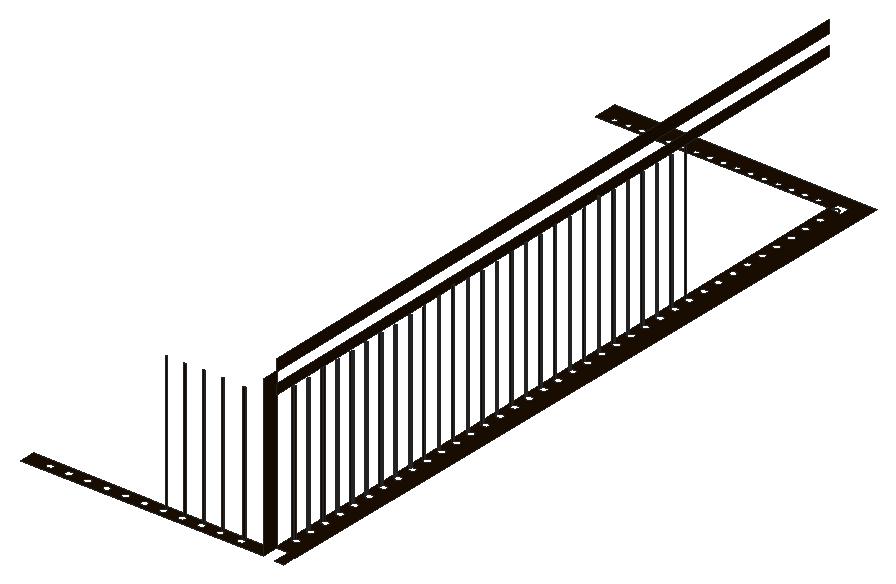
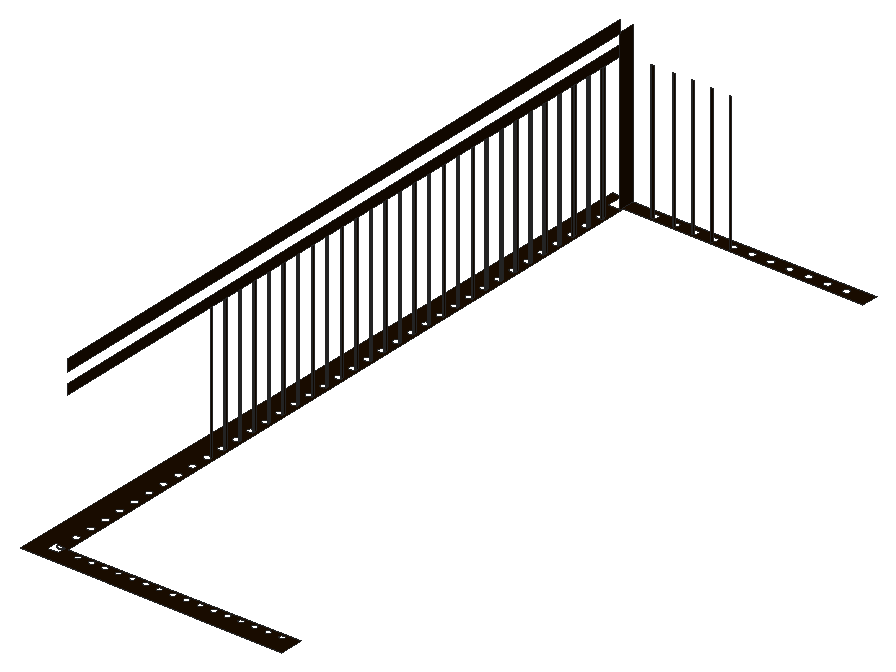
# SketchUp Ruby script. Lengths in inches.
U = 1.inch
M = Sketchup.active_model
def pt(a) = Geom::Point3d.new(a.map { |v| v * U })
def face(e, loops, mat)
  f = e.add_face(loops[0].map { |a| pt(a) })
  loops[1..].each { |l| e.add_face(l.map { |a| pt(a) }).erase! }
  f.material = f.back_material = mat if mat
  f
end
# faces: each face lists its corners as indices into pts; further lists are holes
def faces(e, pts, list, mat = nil) = list.each { |f| face(e, (f[0].is_a?(Array) ? f : [f]).map { |l| l.map { |i| pts[i] } }, mat) }
# xy, xz, yz: faces in a plane at the given z, y or x. An outline is a flat list of corners, or four numbers for a rectangle; further outlines are holes
def ring(l) = l.size == 4 ? [[l[0], l[1]], [l[2], l[1]], [l[2], l[3]], [l[0], l[3]]] : l.each_slice(2).to_a
def flat(e, list, mat, &to3) = list.each { |f| face(e, (f[0].is_a?(Array) ? f : [f]).map { |l| ring(l).map { |u, v| to3.(u, v) } }, mat) }
def xy(e, z, list, mat = nil) = flat(e, list, mat) { |x, y| [x, y, z] }
def xz(e, y, list, mat = nil) = flat(e, list, mat) { |x, z| [x, y, z] }
def yz(e, x, list, mat = nil) = flat(e, list, mat) { |y, z| [x, y, z] }
def lines(e, pts, list) = list.each { |a, b| e.add_line(pt(pts[a]), pt(pts[b])) }
# prism: a flat outline (further loops are holes) pulled along v
def prism(e, loops, v, mat = nil)
  f = face(e, loops, mat); d = Geom::Vector3d.new(v.map { |x| x * U })
  f.pushpull(f.normal.samedirection?(d) ? d.length : -d.length)
end
def box(e, o, s, mat = nil) = prism(e, [[o, [o[0] + s[0], o[1], o[2]], [o[0] + s[0], o[1] + s[1], o[2]], [o[0], o[1] + s[1], o[2]]]], [0, 0, s[2]], mat)
def at(x, y, z, deg = 0) = Geom::Transformation.translation(pt([x, y, z])) * Geom::Transformation.rotation(ORIGIN, Z_AXIS, deg.degrees)
def axes(o, x, y, z) = Geom::Transformation.new([*x, 0, *y, 0, *z, 0, *pt(o).to_a, 1])
def part(name) = M.definitions.add(name)
# library, detail: a bought-in or finely detailed component or shape, given as its bounding box
def library(name, o, s) = part(name).tap { |d| box(d.entities, o, s) }
def detail(e, o, s) = box(e.add_group.entities, o, s)
def put(e, d, t, mat = nil) = e.add_instance(d, t).tap { |i| i.material = mat if mat }
def group(e, t, mat = nil) = e.add_group.tap { |g| g.transformation = t; g.material = mat if mat }.entities
root = M.entities
M.materials.add("[Metal Seamed]1").color = [28, 14, 0]
xy(root,618.25,[[[275.92,67.28,361.97,67.28,361.97,73.28,366.15,73.28,366.15,67.28,369.3125,67.28,369.3125,72.19,369.37,72.19,372.33,325.44,278.88,326.53,278.8125,320.82,278.79,318.92,278.78,318.35,361.23,318.35,361.23,72.29,275.92,73.28],[361.98,317.52,366.15,321.28],[284.2,68.79,283.86,68.83,283.54,68.97,283.27,69.17,283.0625,69.45,282.93,69.76,282.89,70.1,282.93,70.44,283.0625,70.76,283.27,71.03,283.54,71.24,283.86,71.37,284.2,71.41,284.54,71.37,284.86,71.24,285.13,71.03,285.34,70.76,285.47,70.44,285.51,70.1,285.47,69.76,285.34,69.45,285.13,69.17,284.86,68.97,284.54,68.83],[351.89,68.79,351.55,68.83,351.23,68.97,350.96,69.17,350.75,69.45,350.62,69.76,350.58,70.1,350.62,70.44,350.75,70.76,350.96,71.03,351.23,71.24,351.55,71.37,351.89,71.41,352.23,71.37,352.55,71.24,352.82,71.03,353.03,70.76,353.16,70.44,353.2,70.1,353.16,69.76,353.03,69.45,352.82,69.17,352.55,68.97,352.23,68.83],[344.39,68.79,344.05,68.83,343.73,68.97,343.46,69.17,343.25,69.45,343.12,69.76,343.07,70.1,343.12,70.44,343.25,70.76,343.46,71.03,343.73,71.24,344.05,71.37,344.39,71.41,344.73,71.37,345.04,71.24,345.31,71.03,345.52,70.76,345.65,70.44,345.7,70.1,345.65,69.76,345.52,69.45,345.31,69.17,345.04,68.97,344.73,68.83],[337.7,68.79,337.36,68.83,337.04,68.97,336.77,69.17,336.5625,69.45,336.43,69.76,336.39,70.1,336.43,70.44,336.5625,70.76,336.77,71.03,337.04,71.24,337.36,71.37,337.7,71.41,338.04,71.37,338.36,71.24,338.63,71.03,338.84,70.76,338.97,70.44,339.01,70.1,338.97,69.76,338.84,69.45,338.63,69.17,338.36,68.97,338.04,68.83],[331.01,68.79,330.67,68.83,330.36,68.97,330.08,69.17,329.875,69.45,329.74,69.76,329.7,70.1,329.74,70.44,329.875,70.76,330.08,71.03,330.36,71.24,330.67,71.37,331.01,71.41,331.35,71.37,331.67,71.24,331.94,71.03,332.15,70.76,332.28,70.44,332.32,70.1,332.28,69.76,332.15,69.45,331.94,69.17,331.67,68.97,331.35,68.83],[324.32,68.79,323.98,68.83,323.67,68.97,323.4,69.17,323.1875,69.45,323.06,69.76,323.01,70.1,323.06,70.44,323.1875,70.76,323.4,71.03,323.67,71.24,323.98,71.37,324.32,71.41,324.66,71.37,324.98,71.24,325.25,71.03,325.46,70.76,325.59,70.44,325.64,70.1,325.59,69.76,325.46,69.45,325.25,69.17,324.98,68.97,324.66,68.83],[317.64,68.79,317.3,68.83,316.98,68.97,316.71,69.17,316.5,69.45,316.37,69.76,316.32,70.1,316.37,70.44,316.5,70.76,316.71,71.03,316.98,71.24,317.3,71.37,317.64,71.41,317.98,71.37,318.29,71.24,318.56,71.03,318.77,70.76,318.9,70.44,318.95,70.1,318.9,69.76,318.77,69.45,318.56,69.17,318.29,68.97,317.98,68.83],[310.95,68.79,310.61,68.83,310.29,68.97,310.02,69.17,309.8125,69.45,309.68,69.76,309.64,70.1,309.68,70.44,309.8125,70.76,310.02,71.03,310.29,71.24,310.61,71.37,310.95,71.41,311.29,71.37,311.61,71.24,311.88,71.03,312.09,70.76,312.22,70.44,312.26,70.1,312.22,69.76,312.09,69.45,311.88,69.17,311.61,68.97,311.29,68.83],[304.26,68.79,303.92,68.83,303.61,68.97,303.33,69.17,303.125,69.45,302.99,69.76,302.95,70.1,302.99,70.44,303.125,70.76,303.33,71.03,303.61,71.24,303.92,71.37,304.26,71.41,304.6,71.37,304.92,71.24,305.19,71.03,305.4,70.76,305.53,70.44,305.57,70.1,305.53,69.76,305.4,69.45,305.19,69.17,304.92,68.97,304.6,68.83],[297.57,68.79,297.23,68.83,296.92,68.97,296.65,69.17,296.4375,69.45,296.31,69.76,296.26,70.1,296.31,70.44,296.4375,70.76,296.65,71.03,296.92,71.24,297.23,71.37,297.57,71.41,297.91,71.37,298.23,71.24,298.5,71.03,298.71,70.76,298.84,70.44,298.89,70.1,298.84,69.76,298.71,69.45,298.5,69.17,298.23,68.97,297.91,68.83],[290.89,68.79,290.55,68.83,290.23,68.97,289.96,69.17,289.75,69.45,289.62,69.76,289.57,70.1,289.62,70.44,289.75,70.76,289.96,71.03,290.23,71.24,290.55,71.37,290.89,71.41,291.23,71.37,291.54,71.24,291.81,71.03,292.02,70.76,292.15,70.44,292.2,70.1,292.15,69.76,292.02,69.45,291.81,69.17,291.54,68.97,291.23,68.83],[363.55,310.16,363.21,310.25,362.92,310.42,362.67,310.66,362.5,310.96,362.41,311.29,362.41,311.63,362.5,311.96,362.67,312.26,362.91,312.5,363.2,312.67,363.54,312.76,363.88,312.76,364.21,312.68,364.51,312.51,364.75,312.26,364.92,311.97,365.01,311.64,365.01,311.3,364.93,310.96,364.76,310.67,364.51,310.42,364.22,310.25,363.89,310.16],[363.55,303.72,363.21,303.81,362.92,303.98,362.67,304.22,362.5,304.52,362.41,304.85,362.41,305.19,362.5,305.52,362.67,305.82,362.91,306.0625,363.2,306.24,363.54,306.33,363.88,306.33,364.21,306.24,364.51,306.07,364.75,305.83,364.92,305.53,365.01,305.2,365.01,304.86,364.93,304.53,364.76,304.23,364.51,303.99,364.22,303.8125,363.89,303.72],[363.55,297.29,363.21,297.37,362.92,297.54,362.67,297.78,362.5,298.08,362.41,298.41,362.41,298.75,362.5,299.08,362.67,299.38,362.91,299.625,363.2,299.8,363.54,299.89,363.88,299.89,364.21,299.8,364.51,299.63,364.75,299.39,364.92,299.09,365.01,298.76,365.01,298.42,364.93,298.09,364.76,297.79,364.51,297.55,364.22,297.375,363.89,297.29],[363.55,290.85,363.21,290.94,362.92,291.11,362.67,291.35,362.5,291.64,362.41,291.97,362.41,292.32,362.5,292.65,362.67,292.94,362.91,293.1875,363.2,293.36,363.54,293.45,363.88,293.45,364.21,293.36,364.51,293.19,364.75,292.95,364.92,292.66,365.01,292.33,365.01,291.98,364.93,291.65,364.76,291.35,364.51,291.11,364.22,290.9375,363.89,290.85],[363.55,284.41,363.21,284.5,362.92,284.67,362.67,284.91,362.5,285.21,362.41,285.54,362.41,285.88,362.5,286.21,362.67,286.51,362.91,286.75,363.2,286.92,363.54,287.01,363.88,287.01,364.21,286.93,364.51,286.76,364.75,286.51,364.92,286.22,365.01,285.89,365.01,285.55,364.93,285.21,364.76,284.92,364.51,284.67,364.22,284.5,363.89,284.41],[363.55,277.97,363.21,278.06,362.92,278.23,362.67,278.47,362.5,278.77,362.41,279.1,362.41,279.44,362.5,279.77,362.67,280.07,362.91,280.3125,363.2,280.49,363.54,280.58,363.88,280.58,364.21,280.49,364.51,280.32,364.75,280.08,364.92,279.78,365.01,279.45,365.01,279.11,364.93,278.78,364.76,278.48,364.51,278.24,364.22,278.0625,363.89,277.97],[363.55,271.54,363.21,271.62,362.92,271.79,362.67,272.03,362.5,272.33,362.41,272.66,362.41,273,362.5,273.33,362.67,273.63,362.91,273.875,363.2,274.05,363.54,274.14,363.88,274.14,364.21,274.05,364.51,273.88,364.75,273.64,364.92,273.34,365.01,273.01,365.01,272.67,364.93,272.34,364.76,272.04,364.51,271.8,364.22,271.625,363.89,271.54],[363.55,265.1,363.21,265.19,362.92,265.36,362.67,265.6,362.5,265.89,362.41,266.22,362.41,266.57,362.5,266.9,362.67,267.19,362.91,267.4375,363.2,267.61,363.54,267.7,363.88,267.7,364.21,267.61,364.51,267.44,364.75,267.2,364.92,266.91,365.01,266.58,365.01,266.23,364.93,265.9,364.76,265.6,364.51,265.36,364.22,265.1875,363.89,265.1],[363.55,258.66,363.21,258.75,362.92,258.92,362.67,259.16,362.5,259.46,362.41,259.79,362.41,260.13,362.5,260.46,362.67,260.76,362.91,261,363.2,261.17,363.54,261.26,363.88,261.26,364.21,261.18,364.51,261.01,364.75,260.76,364.92,260.47,365.01,260.14,365.01,259.8,364.93,259.46,364.76,259.17,364.51,258.92,364.22,258.75,363.89,258.66],[363.55,252.22,363.21,252.31,362.92,252.48,362.67,252.72,362.5,253.02,362.41,253.35,362.41,253.69,362.5,254.02,362.67,254.32,362.91,254.5625,363.2,254.74,363.54,254.83,363.88,254.83,364.21,254.74,364.51,254.57,364.75,254.33,364.92,254.03,365.01,253.7,365.01,253.36,364.93,253.03,364.76,252.73,364.51,252.49,364.22,252.3125,363.89,252.22],[363.55,245.79,363.21,245.87,362.92,246.04,362.67,246.28,362.5,246.58,362.41,246.91,362.41,247.25,362.5,247.58,362.67,247.88,362.91,248.125,363.2,248.3,363.54,248.39,363.88,248.39,364.21,248.3,364.51,248.13,364.75,247.89,364.92,247.59,365.01,247.26,365.01,246.92,364.93,246.59,364.76,246.29,364.51,246.05,364.22,245.875,363.89,245.79],[363.55,239.35,363.21,239.44,362.92,239.61,362.67,239.85,362.5,240.14,362.41,240.47,362.41,240.82,362.5,241.15,362.67,241.44,362.91,241.6875,363.2,241.86,363.54,241.95,363.88,241.95,364.21,241.86,364.51,241.69,364.75,241.45,364.92,241.16,365.01,240.83,365.01,240.48,364.93,240.15,364.76,239.85,364.51,239.61,364.22,239.4375,363.89,239.35],[363.55,232.91,363.21,233,362.92,233.17,362.67,233.41,362.5,233.71,362.41,234.04,362.41,234.38,362.5,234.71,362.67,235.01,362.91,235.25,363.2,235.42,363.54,235.51,363.88,235.51,364.21,235.43,364.51,235.26,364.75,235.01,364.92,234.72,365.01,234.39,365.01,234.05,364.93,233.71,364.76,233.42,364.51,233.17,364.22,233,363.89,232.91],[363.55,226.47,363.21,226.56,362.92,226.73,362.67,226.97,362.5,227.27,362.41,227.6,362.41,227.94,362.5,228.27,362.67,228.57,362.91,228.8125,363.2,228.99,363.54,229.08,363.88,229.08,364.21,228.99,364.51,228.82,364.75,228.58,364.92,228.28,365.01,227.95,365.01,227.61,364.93,227.28,364.76,226.98,364.51,226.74,364.22,226.5625,363.89,226.47],[363.55,220.04,363.21,220.12,362.92,220.29,362.67,220.53,362.5,220.83,362.41,221.16,362.41,221.5,362.5,221.83,362.67,222.13,362.91,222.375,363.2,222.55,363.54,222.64,363.88,222.64,364.21,222.55,364.51,222.38,364.75,222.14,364.92,221.84,365.01,221.51,365.01,221.17,364.93,220.84,364.76,220.54,364.51,220.3,364.22,220.125,363.89,220.04],[363.55,213.6,363.21,213.69,362.92,213.86,362.67,214.1,362.5,214.39,362.41,214.72,362.41,215.07,362.5,215.4,362.67,215.69,362.91,215.9375,363.2,216.11,363.54,216.2,363.88,216.2,364.21,216.11,364.51,215.94,364.75,215.7,364.92,215.41,365.01,215.08,365.01,214.73,364.93,214.4,364.76,214.1,364.51,213.86,364.22,213.6875,363.89,213.6],[363.55,207.16,363.21,207.25,362.92,207.42,362.67,207.66,362.5,207.96,362.41,208.29,362.41,208.63,362.5,208.96,362.67,209.26,362.91,209.5,363.2,209.67,363.54,209.76,363.88,209.76,364.21,209.68,364.51,209.51,364.75,209.26,364.92,208.97,365.01,208.64,365.01,208.3,364.93,207.96,364.76,207.67,364.51,207.42,364.22,207.25,363.89,207.16],[363.55,200.72,363.21,200.81,362.92,200.98,362.67,201.22,362.5,201.52,362.41,201.85,362.41,202.19,362.5,202.52,362.67,202.82,362.91,203.0625,363.2,203.24,363.54,203.33,363.88,203.33,364.21,203.24,364.51,203.07,364.75,202.83,364.92,202.53,365.01,202.2,365.01,201.86,364.93,201.53,364.76,201.23,364.51,200.99,364.22,200.8125,363.89,200.72],[363.55,194.29,363.21,194.37,362.92,194.54,362.67,194.78,362.5,195.08,362.41,195.41,362.41,195.75,362.5,196.08,362.67,196.38,362.91,196.625,363.2,196.8,363.54,196.89,363.88,196.89,364.21,196.8,364.51,196.63,364.75,196.39,364.92,196.09,365.01,195.76,365.01,195.42,364.93,195.09,364.76,194.79,364.51,194.55,364.22,194.375,363.89,194.29],[363.55,187.85,363.21,187.94,362.92,188.11,362.67,188.35,362.5,188.64,362.41,188.97,362.41,189.32,362.5,189.65,362.67,189.94,362.91,190.1875,363.2,190.36,363.54,190.45,363.88,190.45,364.21,190.36,364.51,190.19,364.75,189.95,364.92,189.66,365.01,189.33,365.01,188.98,364.93,188.65,364.76,188.35,364.51,188.11,364.22,187.9375,363.89,187.85],[363.55,181.41,363.21,181.5,362.92,181.67,362.67,181.91,362.5,182.21,362.41,182.54,362.41,182.88,362.5,183.21,362.67,183.51,362.91,183.75,363.2,183.92,363.54,184.01,363.88,184.01,364.21,183.93,364.51,183.76,364.75,183.51,364.92,183.22,365.01,182.89,365.01,182.55,364.93,182.21,364.76,181.92,364.51,181.67,364.22,181.5,363.89,181.41],[363.55,174.97,363.21,175.06,362.92,175.23,362.67,175.47,362.5,175.77,362.41,176.1,362.41,176.44,362.5,176.77,362.67,177.07,362.91,177.3125,363.2,177.49,363.54,177.58,363.88,177.58,364.21,177.49,364.51,177.32,364.75,177.08,364.92,176.78,365.01,176.45,365.01,176.11,364.93,175.78,364.76,175.48,364.51,175.24,364.22,175.0625,363.89,174.97],[363.55,168.54,363.21,168.62,362.92,168.79,362.67,169.03,362.5,169.33,362.41,169.66,362.41,170,362.5,170.33,362.67,170.63,362.91,170.875,363.2,171.05,363.54,171.14,363.88,171.14,364.21,171.05,364.51,170.88,364.75,170.64,364.92,170.34,365.01,170.01,365.01,169.67,364.93,169.34,364.76,169.04,364.51,168.8,364.22,168.625,363.89,168.54],[363.55,162.1,363.21,162.19,362.92,162.36,362.67,162.6,362.5,162.89,362.41,163.22,362.41,163.57,362.5,163.9,362.67,164.19,362.91,164.4375,363.2,164.61,363.54,164.7,363.88,164.7,364.21,164.61,364.51,164.44,364.75,164.2,364.92,163.91,365.01,163.58,365.01,163.23,364.93,162.9,364.76,162.6,364.51,162.36,364.22,162.1875,363.89,162.1],[363.55,155.66,363.21,155.75,362.92,155.92,362.67,156.16,362.5,156.46,362.41,156.79,362.41,157.13,362.5,157.46,362.67,157.76,362.91,158,363.2,158.17,363.54,158.26,363.88,158.26,364.21,158.18,364.51,158.01,364.75,157.76,364.92,157.47,365.01,157.14,365.01,156.8,364.93,156.46,364.76,156.17,364.51,155.92,364.22,155.75,363.89,155.66],[363.55,149.22,363.21,149.31,362.92,149.48,362.67,149.72,362.5,150.02,362.41,150.35,362.41,150.69,362.5,151.02,362.67,151.32,362.91,151.5625,363.2,151.74,363.54,151.83,363.88,151.83,364.21,151.74,364.51,151.57,364.75,151.33,364.92,151.03,365.01,150.7,365.01,150.36,364.93,150.03,364.76,149.73,364.51,149.49,364.22,149.3125,363.89,149.22],[363.55,142.79,363.21,142.87,362.92,143.04,362.67,143.28,362.5,143.58,362.41,143.91,362.41,144.25,362.5,144.58,362.67,144.88,362.91,145.125,363.2,145.3,363.54,145.39,363.88,145.39,364.21,145.3,364.51,145.13,364.75,144.89,364.92,144.59,365.01,144.26,365.01,143.92,364.93,143.59,364.76,143.29,364.51,143.05,364.22,142.875,363.89,142.79],[363.55,136.35,363.21,136.44,362.92,136.61,362.67,136.85,362.5,137.14,362.41,137.47,362.41,137.82,362.5,138.15,362.67,138.44,362.91,138.6875,363.2,138.86,363.54,138.95,363.88,138.95,364.21,138.86,364.51,138.69,364.75,138.45,364.92,138.16,365.01,137.83,365.01,137.48,364.93,137.15,364.76,136.85,364.51,136.61,364.22,136.4375,363.89,136.35],[363.55,129.91,363.21,130,362.92,130.17,362.67,130.41,362.5,130.71,362.41,131.04,362.41,131.38,362.5,131.71,362.67,132.01,362.91,132.25,363.2,132.42,363.54,132.51,363.88,132.51,364.21,132.43,364.51,132.26,364.75,132.01,364.92,131.72,365.01,131.39,365.01,131.05,364.93,130.71,364.76,130.42,364.51,130.17,364.22,130,363.89,129.91],[363.55,123.47,363.21,123.56,362.92,123.73,362.67,123.97,362.5,124.27,362.41,124.6,362.41,124.94,362.5,125.27,362.67,125.57,362.91,125.8125,363.2,125.99,363.54,126.08,363.88,126.08,364.21,125.99,364.51,125.82,364.75,125.58,364.92,125.28,365.01,124.95,365.01,124.61,364.93,124.28,364.76,123.98,364.51,123.74,364.22,123.5625,363.89,123.47],[363.55,117.04,363.21,117.12,362.92,117.29,362.67,117.53,362.5,117.83,362.41,118.16,362.41,118.5,362.5,118.83,362.67,119.13,362.91,119.375,363.2,119.55,363.54,119.64,363.88,119.64,364.21,119.55,364.51,119.38,364.75,119.14,364.92,118.84,365.01,118.51,365.01,118.17,364.93,117.84,364.76,117.54,364.51,117.3,364.22,117.125,363.89,117.04],[363.55,110.6,363.21,110.69,362.92,110.86,362.67,111.1,362.5,111.39,362.41,111.72,362.41,112.07,362.5,112.4,362.67,112.69,362.91,112.9375,363.2,113.11,363.54,113.2,363.88,113.2,364.21,113.11,364.51,112.94,364.75,112.7,364.92,112.41,365.01,112.08,365.01,111.73,364.93,111.4,364.76,111.1,364.51,110.86,364.22,110.6875,363.89,110.6],[363.55,104.16,363.21,104.25,362.92,104.42,362.67,104.66,362.5,104.96,362.41,105.29,362.41,105.63,362.5,105.96,362.67,106.26,362.91,106.5,363.2,106.67,363.54,106.76,363.88,106.76,364.21,106.68,364.51,106.51,364.75,106.26,364.92,105.97,365.01,105.64,365.01,105.3,364.93,104.96,364.76,104.67,364.51,104.42,364.22,104.25,363.89,104.16],[363.55,97.72,363.21,97.81,362.92,97.98,362.67,98.22,362.5,98.52,362.41,98.85,362.41,99.19,362.5,99.52,362.67,99.82,362.91,100.0625,363.2,100.24,363.54,100.33,363.88,100.33,364.21,100.24,364.51,100.07,364.75,99.83,364.92,99.53,365.01,99.2,365.01,98.86,364.93,98.53,364.76,98.23,364.51,97.99,364.22,97.8125,363.89,97.72],[363.55,91.29,363.21,91.37,362.92,91.54,362.67,91.78,362.5,92.08,362.41,92.41,362.41,92.75,362.5,93.08,362.67,93.38,362.91,93.625,363.2,93.8,363.54,93.89,363.88,93.89,364.21,93.8,364.51,93.63,364.75,93.39,364.92,93.09,365.01,92.76,365.01,92.42,364.93,92.09,364.76,91.79,364.51,91.55,364.22,91.375,363.89,91.29],[363.55,84.85,363.21,84.94,362.92,85.11,362.67,85.35,362.5,85.64,362.41,85.97,362.41,86.32,362.5,86.65,362.67,86.94,362.91,87.1875,363.2,87.36,363.54,87.45,363.88,87.45,364.21,87.36,364.51,87.19,364.75,86.95,364.92,86.66,365.01,86.33,365.01,85.98,364.93,85.65,364.76,85.35,364.51,85.11,364.22,84.9375,363.89,84.85],[363.55,78.41,363.21,78.5,362.92,78.67,362.67,78.91,362.5,79.21,362.41,79.54,362.41,79.88,362.5,80.21,362.67,80.51,362.91,80.75,363.2,80.92,363.54,81.01,363.88,81.01,364.21,80.93,364.51,80.76,364.75,80.51,364.92,80.22,365.01,79.89,365.01,79.55,364.93,79.21,364.76,78.92,364.51,78.67,364.22,78.5,363.89,78.41],[356.27,318.74,355.98,318.8125,355.73,318.95,355.51,319.15,355.36,319.4,355.28,319.6875,355.27,319.98,355.34,320.27,355.48,320.52,355.68,320.74,355.93,320.89,356.21,320.97,356.5,320.98,356.79,320.91,357.05,320.77,357.26,320.57,357.41,320.32,357.5,320.04,357.51,319.74,357.4375,319.46,357.3,319.2,357.09,318.99,356.84,318.83,356.5625,318.75],[284.08,318.74,283.8,318.8125,283.54,318.95,283.32,319.15,283.17,319.4,283.09,319.6875,283.08,319.98,283.15,320.27,283.29,320.52,283.49,320.74,283.74,320.89,284.02,320.97,284.32,320.98,284.6,320.91,284.86,320.77,285.07,320.57,285.23,320.32,285.31,320.04,285.32,319.74,285.25,319.46,285.11,319.2,284.91,318.99,284.66,318.83,284.375,318.75],[288.89,318.74,288.61,318.8125,288.35,318.95,288.14,319.15,287.98,319.4,287.9,319.6875,287.89,319.98,287.96,320.27,288.1,320.52,288.3,320.74,288.55,320.89,288.84,320.97,289.13,320.98,289.41,320.91,289.67,320.77,289.89,320.57,290.04,320.32,290.12,320.04,290.13,319.74,290.0625,319.46,289.92,319.2,289.72,318.99,289.47,318.83,289.1875,318.75],[293.71,318.74,293.42,318.8125,293.16,318.95,292.95,319.15,292.8,319.4,292.71,319.6875,292.71,319.98,292.77,320.27,292.91,320.52,293.12,320.74,293.37,320.89,293.65,320.97,293.94,320.98,294.23,320.91,294.49,320.77,294.7,320.57,294.85,320.32,294.94,320.04,294.94,319.74,294.875,319.46,294.73,319.2,294.53,318.99,294.28,318.83,294,318.75],[298.52,318.74,298.23,318.8125,297.98,318.95,297.76,319.15,297.61,319.4,297.53,319.6875,297.52,319.98,297.59,320.27,297.73,320.52,297.93,320.74,298.18,320.89,298.46,320.97,298.75,320.98,299.04,320.91,299.3,320.77,299.51,320.57,299.66,320.32,299.75,320.04,299.76,319.74,299.6875,319.46,299.55,319.2,299.34,318.99,299.09,318.83,298.8125,318.75],[303.33,318.74,303.05,318.8125,302.79,318.95,302.57,319.15,302.42,319.4,302.34,319.6875,302.33,319.98,302.4,320.27,302.54,320.52,302.74,320.74,302.99,320.89,303.27,320.97,303.57,320.98,303.85,320.91,304.11,320.77,304.32,320.57,304.48,320.32,304.56,320.04,304.57,319.74,304.5,319.46,304.36,319.2,304.16,318.99,303.91,318.83,303.625,318.75],[308.14,318.74,307.86,318.8125,307.6,318.95,307.39,319.15,307.23,319.4,307.15,319.6875,307.14,319.98,307.21,320.27,307.35,320.52,307.55,320.74,307.8,320.89,308.09,320.97,308.38,320.98,308.66,320.91,308.92,320.77,309.14,320.57,309.29,320.32,309.37,320.04,309.38,319.74,309.3125,319.46,309.17,319.2,308.97,318.99,308.72,318.83,308.4375,318.75],[312.96,318.74,312.67,318.8125,312.41,318.95,312.2,319.15,312.05,319.4,311.96,319.6875,311.96,319.98,312.02,320.27,312.16,320.52,312.37,320.74,312.62,320.89,312.9,320.97,313.19,320.98,313.48,320.91,313.74,320.77,313.95,320.57,314.1,320.32,314.19,320.04,314.19,319.74,314.125,319.46,313.98,319.2,313.78,318.99,313.53,318.83,313.25,318.75],[317.77,318.74,317.48,318.8125,317.23,318.95,317.01,319.15,316.86,319.4,316.78,319.6875,316.77,319.98,316.84,320.27,316.98,320.52,317.18,320.74,317.43,320.89,317.71,320.97,318,320.98,318.29,320.91,318.55,320.77,318.76,320.57,318.91,320.32,319,320.04,319.01,319.74,318.9375,319.46,318.8,319.2,318.59,318.99,318.34,318.83,318.0625,318.75],[322.58,318.74,322.3,318.8125,322.04,318.95,321.82,319.15,321.67,319.4,321.59,319.6875,321.58,319.98,321.65,320.27,321.79,320.52,321.99,320.74,322.24,320.89,322.52,320.97,322.82,320.98,323.1,320.91,323.36,320.77,323.57,320.57,323.73,320.32,323.81,320.04,323.82,319.74,323.75,319.46,323.61,319.2,323.41,318.99,323.16,318.83,322.875,318.75],[327.39,318.74,327.11,318.8125,326.85,318.95,326.64,319.15,326.48,319.4,326.4,319.6875,326.39,319.98,326.46,320.27,326.6,320.52,326.8,320.74,327.05,320.89,327.34,320.97,327.63,320.98,327.91,320.91,328.17,320.77,328.39,320.57,328.54,320.32,328.62,320.04,328.63,319.74,328.5625,319.46,328.42,319.2,328.22,318.99,327.97,318.83,327.6875,318.75],[332.21,318.74,331.92,318.8125,331.66,318.95,331.45,319.15,331.3,319.4,331.21,319.6875,331.21,319.98,331.27,320.27,331.41,320.52,331.62,320.74,331.87,320.89,332.15,320.97,332.44,320.98,332.73,320.91,332.99,320.77,333.2,320.57,333.35,320.32,333.44,320.04,333.44,319.74,333.375,319.46,333.23,319.2,333.03,318.99,332.78,318.83,332.5,318.75],[337.02,318.74,336.73,318.8125,336.48,318.95,336.26,319.15,336.11,319.4,336.03,319.6875,336.02,319.98,336.09,320.27,336.23,320.52,336.43,320.74,336.68,320.89,336.96,320.97,337.25,320.98,337.54,320.91,337.8,320.77,338.01,320.57,338.16,320.32,338.25,320.04,338.26,319.74,338.1875,319.46,338.05,319.2,337.84,318.99,337.59,318.83,337.3125,318.75],[341.83,318.74,341.55,318.8125,341.29,318.95,341.07,319.15,340.92,319.4,340.84,319.6875,340.83,319.98,340.9,320.27,341.04,320.52,341.24,320.74,341.49,320.89,341.77,320.97,342.07,320.98,342.35,320.91,342.61,320.77,342.82,320.57,342.98,320.32,343.06,320.04,343.07,319.74,343,319.46,342.86,319.2,342.66,318.99,342.41,318.83,342.125,318.75],[346.64,318.74,346.36,318.8125,346.1,318.95,345.89,319.15,345.73,319.4,345.65,319.6875,345.64,319.98,345.71,320.27,345.85,320.52,346.05,320.74,346.3,320.89,346.59,320.97,346.88,320.98,347.16,320.91,347.42,320.77,347.64,320.57,347.79,320.32,347.87,320.04,347.88,319.74,347.8125,319.46,347.67,319.2,347.47,318.99,347.22,318.83,346.9375,318.75],[351.46,318.74,351.17,318.8125,350.91,318.95,350.7,319.15,350.55,319.4,350.46,319.6875,350.46,319.98,350.52,320.27,350.66,320.52,350.87,320.74,351.12,320.89,351.4,320.97,351.69,320.98,351.98,320.91,352.24,320.77,352.45,320.57,352.6,320.32,352.69,320.04,352.69,319.74,352.625,319.46,352.48,319.2,352.28,318.99,352.03,318.83,351.75,318.75],[362.47,317.52,362.41,317.72,362.41,318.07,362.5,318.4,362.67,318.69,362.91,318.9375,363.2,319.11,363.54,319.2,363.88,319.2,364.21,319.11,364.51,318.94,364.75,318.7,364.92,318.41,365.01,318.08,365.01,317.73,364.96,317.52]]],"[Metal Seamed]1")
xz(root,73.28,[[361.97,666.66,361.98,670.37]])
yz(root,361.97,[[67.28,618.25,73.28,674.375],[73.28,674.05,317.52,678.3125]],"[Metal Seamed]1")
yz(root,361.98,[[73.28,666.66,317.52,670.37]],"[Metal Seamed]1")
yz(root,362.41,[[79.54,618.25,79.88,666.66],[85.97,618.25,86.32,666.5625],[92.41,618.25,92.75,666.9375],[98.85,618.25,99.19,666.66],[105.29,618.25,105.63,666.66],
  [111.72,618.25,112.07,666.66],[118.16,618.25,118.5,666.66],[124.6,618.25,124.94,666.375],[131.04,618.25,131.38,666.66],[137.47,618.25,137.82,666.66],
  [143.91,618.25,144.25,667.125],[150.35,618.25,150.69,667.9375],[156.79,618.25,157.13,666.8125],[163.22,618.25,163.57,666.66],[169.66,618.25,170,666.66],
  [176.1,618.25,176.44,667],[182.54,618.25,182.88,667.25],[188.97,618.25,189.32,666.66],[195.41,618.25,195.75,667.125],[201.85,618.25,202.19,666.8125],
  [208.29,618.25,208.63,666.66],[214.72,618.25,215.07,667.8125],[221.16,618.25,221.5,666.75],[227.6,618.25,227.94,666.75],[234.04,618.25,234.38,666.9375],
  [240.47,618.25,240.82,666.66],[246.91,618.25,247.25,666.625]],"[Metal Seamed]1")
p = [[352.55,71.24,618.25],[352.23,71.37,618.25],[352.23,71.37,666.66],[352.55,71.24,666.66],[324.32,71.41,618.25],[323.98,71.37,618.25],
  [323.98,71.37,666.66],[324.32,71.41,666.66],[324.66,71.37,618.25],[324.66,71.37,666.66],[331.01,71.41,618.25],[330.67,71.37,618.25],
  [330.67,71.37,666.66],[331.01,71.41,666.66],[331.35,71.37,618.25],[331.35,71.37,666.66],[337.7,71.41,618.25],[337.36,71.37,618.25],
  [337.36,71.37,666.9375],[337.7,71.41,666.9375],[338.04,71.37,618.25],[338.04,71.37,666.9375],[344.39,71.41,618.25],[344.05,71.37,618.25],
  [344.05,71.37,666.8125],[344.39,71.41,666.8125],[344.73,71.37,618.25],[344.73,71.37,666.8125],[351.89,71.41,618.25],[351.55,71.37,618.25],
  [351.55,71.37,666.66],[351.89,71.41,666.66],[362.41,79.54,618.25],[362.5,79.21,618.25],[362.5,79.21,666.66],[362.41,79.54,666.66],
  [362.5,80.21,618.25],[362.41,79.88,618.25],[362.41,79.88,666.66],[362.5,80.21,666.66],[362.67,80.51,618.25],[362.67,80.51,666.66],
  [362.41,85.97,618.25],[362.5,85.64,618.25],[362.5,85.64,666.5625],[362.41,85.97,666.5625],[362.5,86.65,618.25],[362.41,86.32,618.25],
  [362.41,86.32,666.5625],[362.5,86.65,666.5625],[362.67,86.94,618.25],[362.67,86.94,666.5625],[362.41,92.41,618.25],[362.5,92.08,618.25],
  [362.5,92.08,666.9375],[362.41,92.41,666.9375],[362.5,93.08,618.25],[362.41,92.75,618.25],[362.41,92.75,666.9375],[362.5,93.08,666.9375],
  [362.67,93.38,618.25],[362.67,93.38,666.9375],[362.41,98.85,618.25],[362.5,98.52,618.25],[362.5,98.52,666.66],[362.41,98.85,666.66],
  [362.5,99.52,618.25],[362.41,99.19,618.25],[362.41,99.19,666.66],[362.5,99.52,666.66],[362.67,99.82,618.25],[362.67,99.82,666.66],
  [362.41,105.29,618.25],[362.5,104.96,618.25],[362.5,104.96,666.66],[362.41,105.29,666.66],[362.5,105.96,618.25],[362.41,105.63,618.25],
  [362.41,105.63,666.66],[362.5,105.96,666.66],[362.67,106.26,618.25],[362.67,106.26,666.66],[362.41,111.72,618.25],[362.5,111.39,618.25],
  [362.5,111.39,666.66],[362.41,111.72,666.66],[362.5,112.4,618.25],[362.41,112.07,618.25],[362.41,112.07,666.66],[362.5,112.4,666.66],
  [362.67,112.69,618.25],[362.67,112.69,666.66],[362.41,118.16,618.25],[362.5,117.83,618.25],[362.5,117.83,666.66],[362.41,118.16,666.66],
  [362.5,118.83,618.25],[362.41,118.5,618.25],[362.41,118.5,666.66],[362.5,118.83,666.66],[362.67,119.13,618.25],[362.67,119.13,666.66],
  [362.41,124.6,618.25],[362.5,124.27,618.25],[362.5,124.27,666.375],[362.41,124.6,666.375],[362.5,125.27,618.25],[362.41,124.94,618.25],
  [362.41,124.94,666.375],[362.5,125.27,666.375],[362.67,125.57,618.25],[362.67,125.57,666.375],[362.41,131.04,618.25],[362.5,130.71,618.25],
  [362.5,130.71,666.66],[362.41,131.04,666.66],[362.5,131.71,618.25],[362.41,131.38,618.25],[362.41,131.38,666.66],[362.5,131.71,666.66],
  [362.67,132.01,618.25],[362.67,132.01,666.66],[362.41,137.47,618.25],[362.5,137.14,618.25],[362.5,137.14,666.66],[362.41,137.47,666.66],
  [362.5,138.15,618.25],[362.41,137.82,618.25],[362.41,137.82,666.66],[362.5,138.15,666.66],[362.41,143.91,618.25],[362.5,143.58,618.25],
  [362.5,143.58,667.125],[362.41,143.91,667.125],[362.5,144.58,618.25],[362.41,144.25,618.25],[362.41,144.25,667.125],[362.5,144.58,667.125],
  [362.41,150.35,618.25],[362.5,150.02,618.25],[362.5,150.02,667.9375],[362.41,150.35,667.9375],[362.5,151.02,618.25],[362.41,150.69,618.25],
  [362.41,150.69,667.9375],[362.5,151.02,667.9375],[362.41,156.79,618.25],[362.5,156.46,618.25],[362.5,156.46,666.8125],[362.41,156.79,666.8125],
  [362.5,157.46,618.25],[362.41,157.13,618.25],[362.41,157.13,666.8125],[362.5,157.46,666.8125],[362.41,163.22,618.25],[362.5,162.89,618.25],
  [362.5,162.89,666.66],[362.41,163.22,666.66],[362.5,163.9,618.25],[362.41,163.57,618.25],[362.41,163.57,666.66],[362.5,163.9,666.66],
  [362.41,169.66,618.25],[362.5,169.33,618.25],[362.5,169.33,666.66],[362.41,169.66,666.66],[362.5,170.33,618.25],[362.41,170,618.25],
  [362.41,170,666.66],[362.5,170.33,666.66],[362.41,176.1,618.25],[362.5,175.77,618.25],[362.5,175.77,667],[362.41,176.1,667],
  [362.5,176.77,618.25],[362.41,176.44,618.25],[362.41,176.44,667],[362.5,176.77,667],[362.41,182.54,618.25],[362.5,182.21,618.25],
  [362.5,182.21,667.25],[362.41,182.54,667.25],[362.5,183.21,618.25],[362.41,182.88,618.25],[362.41,182.88,667.25],[362.5,183.21,667.25],
  [362.41,188.97,618.25],[362.5,188.64,618.25],[362.5,188.64,666.66],[362.41,188.97,666.66],[362.5,189.65,618.25],[362.41,189.32,618.25],
  [362.41,189.32,666.66],[362.5,189.65,666.66],[362.41,195.41,618.25],[362.5,195.08,618.25],[362.5,195.08,667.125],[362.41,195.41,667.125],
  [362.5,196.08,618.25],[362.41,195.75,618.25],[362.41,195.75,667.125],[362.5,196.08,667.125],[362.41,201.85,618.25],[362.5,201.52,618.25],
  [362.5,201.52,666.8125],[362.41,201.85,666.8125],[362.5,202.52,618.25],[362.41,202.19,618.25],[362.41,202.19,666.8125],[362.5,202.52,666.8125],
  [362.41,208.29,618.25],[362.5,207.96,618.25],[362.5,207.96,666.66],[362.41,208.29,666.66],[362.5,208.96,618.25],[362.41,208.63,618.25],
  [362.41,208.63,666.66],[362.5,208.96,666.66],[362.41,214.72,618.25],[362.5,214.39,618.25],[362.5,214.39,667.8125],[362.41,214.72,667.8125],
  [362.5,215.4,618.25],[362.41,215.07,618.25],[362.41,215.07,667.8125],[362.5,215.4,667.8125],[362.41,221.16,618.25],[362.5,220.83,618.25],
  [362.5,220.83,666.75],[362.41,221.16,666.75],[362.5,221.83,618.25],[362.41,221.5,618.25],[362.41,221.5,666.75],[362.5,221.83,666.75],
  [362.41,227.6,618.25],[362.5,227.27,618.25],[362.5,227.27,666.75],[362.41,227.6,666.75],[362.5,228.27,618.25],[362.41,227.94,618.25],
  [362.41,227.94,666.75],[362.5,228.27,666.75],[362.41,234.04,618.25],[362.5,233.71,618.25],[362.5,233.71,666.9375],[362.41,234.04,666.9375],
  [362.5,234.71,618.25],[362.41,234.38,618.25],[362.41,234.38,666.9375],[362.5,234.71,666.9375],[362.41,240.47,618.25],[362.5,240.14,618.25],
  [362.5,240.14,666.66],[362.41,240.47,666.66],[362.5,241.15,618.25],[362.41,240.82,618.25],[362.41,240.82,666.66],[362.5,241.15,666.66],
  [362.41,246.91,618.25],[362.5,246.58,618.25],[362.5,246.58,666.625],[362.41,246.91,666.625],[362.5,247.58,618.25],[362.41,247.25,618.25],
  [362.41,247.25,666.625],[362.5,247.58,666.625],[362.41,253.35,618.25],[362.5,253.02,618.25],[362.5,253.02,667],[362.41,253.35,667]]
faces(root,p,[[0,1,2,3],[4,5,6,7],[8,4,7,9],[10,11,12,13],[14,10,13,15],[16,17,18,19],[20,16,19,21],[22,23,24,25],
  [26,22,25,27],[28,29,30,31],[1,28,31,2],[32,33,34,35],[36,37,38,39],[40,36,39,41],[42,43,44,45],[46,47,48,49],
  [50,46,49,51],[52,53,54,55],[56,57,58,59],[60,56,59,61],[62,63,64,65],[66,67,68,69],[70,66,69,71],[72,73,74,75],
  [76,77,78,79],[80,76,79,81],[82,83,84,85],[86,87,88,89],[90,86,89,91],[92,93,94,95],[96,97,98,99],[100,96,99,101],
  [102,103,104,105],[106,107,108,109],[110,106,109,111],[112,113,114,115],[116,117,118,119],[120,116,119,121],[122,123,124,125],[126,127,128,129],
  [130,131,132,133],[134,135,136,137],[138,139,140,141],[142,143,144,145],[146,147,148,149],[150,151,152,153],[154,155,156,157],[158,159,160,161],
  [162,163,164,165],[166,167,168,169],[170,171,172,173],[174,175,176,177],[178,179,180,181],[182,183,184,185],[186,187,188,189],[190,191,192,193],
  [194,195,196,197],[198,199,200,201],[202,203,204,205],[206,207,208,209],[210,211,212,213],[214,215,216,217],[218,219,220,221],[222,223,224,225],
  [226,227,228,229],[230,231,232,233],[234,235,236,237],[238,239,240,241],[242,243,244,245],[246,247,248,249],[250,251,252,253],[254,255,256,257],
  [258,259,260,261],[262,263,264,265],[266,267,268,269]],"[Metal Seamed]1")
